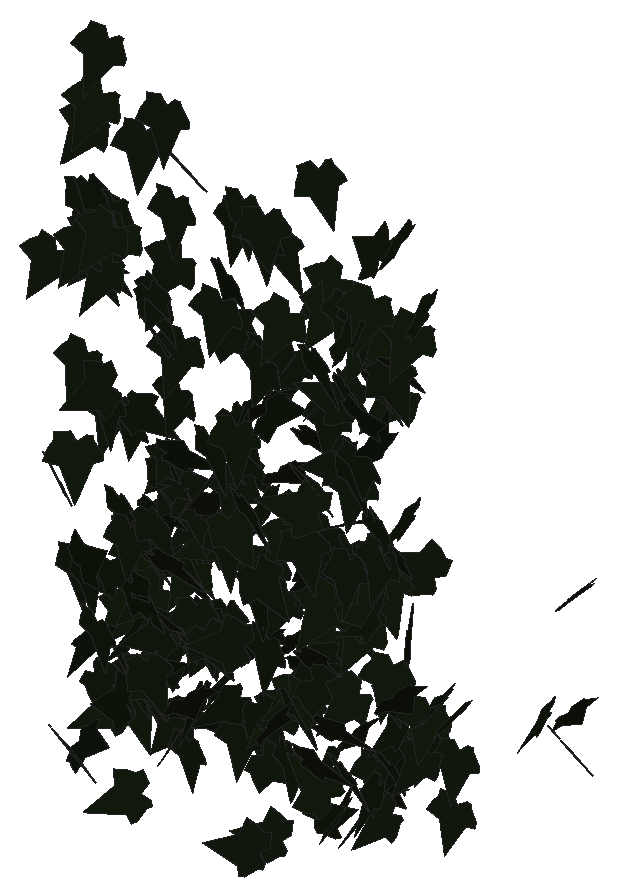
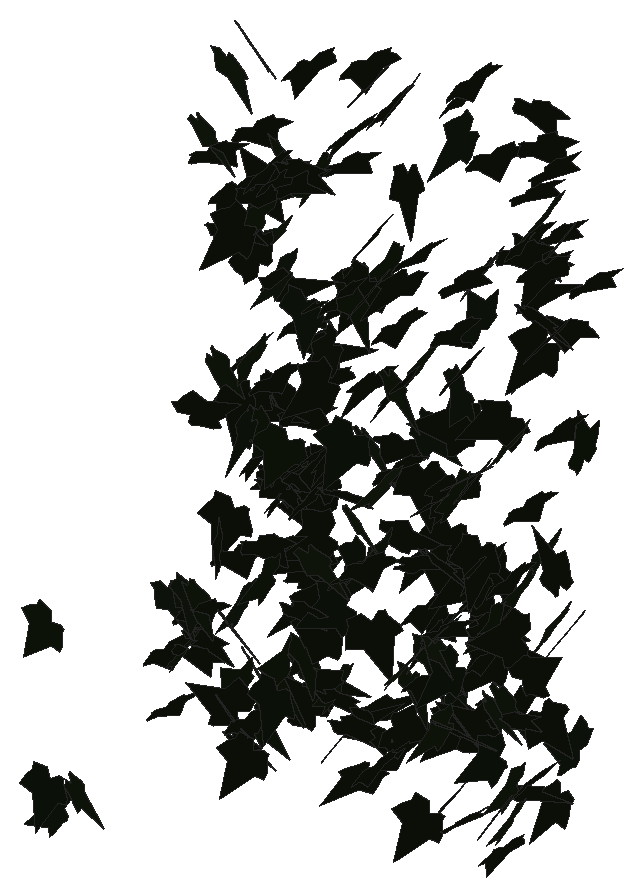
# SketchUp Ruby script. Lengths in inches.
U = 1.inch
M = Sketchup.active_model
def pt(a) = Geom::Point3d.new(a.map { |v| v * U })
def face(e, loops, mat)
  f = e.add_face(loops[0].map { |a| pt(a) })
  loops[1..].each { |l| e.add_face(l.map { |a| pt(a) }).erase! }
  f.material = f.back_material = mat if mat
  f
end
# faces: each face lists its corners as indices into pts; further lists are holes
def faces(e, pts, list, mat = nil) = list.each { |f| face(e, (f[0].is_a?(Array) ? f : [f]).map { |l| l.map { |i| pts[i] } }, mat) }
# xy, xz, yz: faces in a plane at the given z, y or x. An outline is a flat list of corners, or four numbers for a rectangle; further outlines are holes
def ring(l) = l.size == 4 ? [[l[0], l[1]], [l[2], l[1]], [l[2], l[3]], [l[0], l[3]]] : l.each_slice(2).to_a
def flat(e, list, mat, &to3) = list.each { |f| face(e, (f[0].is_a?(Array) ? f : [f]).map { |l| ring(l).map { |u, v| to3.(u, v) } }, mat) }
def xy(e, z, list, mat = nil) = flat(e, list, mat) { |x, y| [x, y, z] }
def xz(e, y, list, mat = nil) = flat(e, list, mat) { |x, z| [x, y, z] }
def yz(e, x, list, mat = nil) = flat(e, list, mat) { |y, z| [x, y, z] }
def lines(e, pts, list) = list.each { |a, b| e.add_line(pt(pts[a]), pt(pts[b])) }
# prism: a flat outline (further loops are holes) pulled along v
def prism(e, loops, v, mat = nil)
  f = face(e, loops, mat); d = Geom::Vector3d.new(v.map { |x| x * U })
  f.pushpull(f.normal.samedirection?(d) ? d.length : -d.length)
end
def box(e, o, s, mat = nil) = prism(e, [[o, [o[0] + s[0], o[1], o[2]], [o[0] + s[0], o[1] + s[1], o[2]], [o[0], o[1] + s[1], o[2]]]], [0, 0, s[2]], mat)
def at(x, y, z, deg = 0) = Geom::Transformation.translation(pt([x, y, z])) * Geom::Transformation.rotation(ORIGIN, Z_AXIS, deg.degrees)
def axes(o, x, y, z) = Geom::Transformation.new([*x, 0, *y, 0, *z, 0, *pt(o).to_a, 1])
def part(name) = M.definitions.add(name)
# library, detail: a bought-in or finely detailed component or shape, given as its bounding box
def library(name, o, s) = part(name).tap { |d| box(d.entities, o, s) }
def detail(e, o, s) = box(e.add_group.entities, o, s)
def put(e, d, t, mat = nil) = e.add_instance(d, t).tap { |i| i.material = mat if mat }
def group(e, t, mat = nil) = e.add_group.tap { |g| g.transformation = t; g.material = mat if mat }.entities
root = M.entities
M.materials.add("efeu1").color = [18, 25, 13]
c1 = part("ivyleaf_9")
p = [[1.54,2.16,1.25],[1.36,2.04,1.19],[-0.21,0.99,0.68],[-0.71,1.11,0.82],[-0.85,0.86,0.67],[-0.8,0.17,0.21],
  [-0.9,-0.01,0.1],[-0.67,-0.16,-0.02],[-0.08,-0.08,-0.05],[-0.03,-0.6,-0.4],[0.65,-0.88,-0.66],[0.83,-0.6,-0.49],
  [1.29,-0.42,-0.43],[1.8125,-0.07,-0.26],[1.21,0.44,0.15]]
faces(c1.entities,p,[[0,1,2,3,4,5,6,7,8,9,10,11,12,13,14]],"efeu1")
put(root,c1,axes([626.05,112.71,371.45],[-0.67145,-1.20045,0.4815],[-0.06051,-0.51277,-1.36278],[1.292,-0.64789,0.18641]))
put(root,c1,axes([625.96,116.39,361.48],[-0.4037,-1.34636,0.39865],[-0.06914,-0.39523,-1.40485],[1.40244,-0.40704,0.04549]))
put(root,c1,axes([625.64,121.35,333.53],[0.81653,-1.05267,-0.13594],[-0.05536,0.12904,-1.33177],[1.05997,0.81765,0.03517]))
put(root,c1,axes([625.7,117.2,369.35],[0.70417,-1.21921,-0.41464],[-0.01473,0.46492,-1.39208],[1.2877,0.67203,0.21082]))
put(root,c1,axes([627.29,117.98,342.52],[0.198,-0.141,1.37987],[-1.18466,0.70779,0.24232],[-0.72144,-1.20094,-0.01919]))
put(root,c1,axes([625.77,115.38,345.34],[0.39319,-1.37533,0.27106],[0.07663,-0.26001,-1.43043],[1.39969,0.40058,0.00217]))
put(root,c1,axes([626.96,116.38,339.04],[-0.2335,0.83704,-1.05981],[0.22412,-1.03661,-0.86809],[-1.33177,-0.3212,0.03973]))
put(root,c1,axes([626.17,117.28,368.65],[1.39761,0.45178,-0.09469],[-0.09171,-0.02413,-1.46881],[-0.45239,1.40061,0.00524]))
put(root,c1,axes([626.47,118.94,356.64],[-0.34395,-1.37252,0.18283],[-0.05405,-0.17494,-1.41493],[1.38359,-0.34803,-0.00983]))
put(root,c1,axes([626.31,121.45,331.08],[0.23264,-1.24833,-0.40414],[0.02751,0.415,-1.26602],[1.31184,0.21267,0.09822]))
put(root,c1,axes([627.52,117.14,370.7],[-1.4735,-0.05512,-0.05772],[0.0613,-0.09832,-1.4711],[0.0511,-1.47135,0.10047]))
put(root,c1,axes([627.05,117.35,387.1],[-1.22917,-0.72135,-0.37924],[0.32497,0.19554,-1.4252],[0.74737,-1.2714,-0.00403]))
put(root,c1,axes([626.3,117.21,335.16],[0.83566,-0.82721,-0.74649],[-0.12031,0.86066,-1.08841],[1.10772,0.71753,0.44493]))
put(root,c1,axes([626.32,120.25,335.4375],[1.06575,-0.85983,-0.0985],[-0.07346,0.06581,-1.36935],[0.86233,1.06827,0.00508]))
put(root,c1,axes([627.13,115.77,381.24],[-0.65135,-1.15831,0.65192],[-0.18119,-0.64184,-1.32142],[1.31676,-0.66129,0.14065]))
put(root,c1,axes([626.42,115.38,375.57],[0.58659,-1.39175,0.06191],[0.02447,-0.05687,-1.51032],[1.39292,0.5871,0.00046]))
put(root,c1,axes([626.68,116.37,374.22],[0.14066,-1.15782,-0.88511],[-0.07596,0.88219,-1.16607],[1.4554,0.15794,0.02468]))
put(root,c1,axes([627.53,119.82,340.03],[-1.08754,-0.82835,0.23481],[-0.04887,-0.31829,-1.34921],[0.8596,-1.0661,0.22037]))
put(root,c1,axes([627.47,113.97,331.47],[-0.03926,0.02081,-1.39293],[-0.76709,1.16288,0.03899],[1.16287,0.7678,-0.0213]))
put(root,c1,axes([626.71,121.72,333.64],[0.58672,-1.21149,-0.08961],[-0.05131,0.07471,-1.34602],[1.21372,0.5888,-0.01359]))
put(root,c1,axes([626.27,119.85,346.82],[1.18693,-0.31127,0.79352],[0.75843,-0.23523,-1.22671],[0.38903,1.40824,-0.02951]))
put(root,c1,axes([627.62,116,383.38],[-1.02712,-1.1019,0.00701],[-0.02789,0.01642,-1.50604],[1.10157,-1.02702,-0.0316]))
put(root,c1,axes([628.29,117.54,333.05],[-1.1996,-0.27111,0.6453],[-0.54996,-0.42696,-1.20174],[0.43296,-1.2935,0.26142]))
put(root,c1,axes([628.3,120.58,341.22],[-1.15049,0.45272,-0.54823],[0.43215,-0.38285,-1.22304],[-0.56459,-1.21557,0.18102]))
put(root,c1,axes([627.27,114.84,345.05],[0.37798,-1.26334,0.48366],[0.14913,-0.46021,-1.31864],[1.34452,0.4062,0.01029]))
put(root,c1,axes([627.37,118.41,349.22],[0.64063,-1.21051,0.35995],[0.16692,-0.31891,-1.36958],[1.25181,0.66202,-0.00158]))
put(root,c1,axes([628.26,115.17,372.93],[-0.69581,-1.09577,0.67655],[-0.16852,-0.6849,-1.28261],[1.27672,-0.68759,0.19942]))
put(root,c1,axes([627.93,120.16,337.06],[1.29444,-0.24286,0.25292],[0.24253,-0.07849,-1.31664],[0.25324,1.31658,-0.03184]))
put(root,c1,axes([628.16,114.17,377.01],[0.90407,-1.16045,-0.26707],[-0.08156,0.27419,-1.46747],[1.18799,0.90194,0.1025]))
put(root,c1,axes([628.84,119.23,345.84],[-0.71,-1.10406,-0.33576],[0.36371,0.16003,-1.29534],[1.09517,-0.76891,0.21251]))
put(root,c1,axes([630.01,117.11,340.04],[-1.02088,0.95691,-0.16624],[0.10553,-0.13047,-1.39906],[-0.9655,-1.02607,0.02286]))
put(root,c1,axes([629.05,115.66,375.1],[-0.11695,-1.44613,0.25942],[-0.03601,-0.25734,-1.45078],[1.46878,-0.12146,-0.01491]))
put(root,c1,axes([629.54,112.14,373.77],[-0.67362,-1.19407,0.51458],[-0.08169,-0.53952,-1.35889],[1.29765,-0.65381,0.18157]))
put(root,c1,axes([628.52,110.67,333.26],[0.84672,-0.92304,0.76005],[0.58924,-0.48827,-1.24941],[1.04043,1.02772,0.08904]))
put(root,c1,axes([628.84,112.33,347.07],[-0.16438,0.13905,1.47625],[0.91408,-1.15999,0.21104],[1.16752,0.92777,0.04261]))
put(root,c1,axes([628.95,109.42,355.53],[-0.027,-0.57991,1.37103],[0.55583,-1.27601,-0.52878],[1.38097,0.50224,0.23963]))
put(root,c1,axes([629.24,119.5625,344.44],[0.16291,-1.35705,-0.09852],[-0.01392,0.09755,-1.36679],[1.36055,0.16349,-0.00219]))
put(root,c1,axes([629.04,118.39,346.44],[1.20901,-0.69536,-0.09625],[-0.04936,0.10701,-1.39306],[0.70025,1.20811,0.06799]))
put(root,c1,axes([630.15,115.24,373.71],[-0.90624,-1.171,0.03617],[-0.00741,-0.04,-1.48059],[1.17153,-0.90608,0.01862]))
put(root,c1,axes([630.01,116.43,348.6],[-0.04433,-1.39838,0.16525],[-0.01018,-0.16501,-1.39908],[1.40808,-0.04522,-0.00491]))
put(root,c1,axes([631.61,121.4,338.7],[-1.2008,0.3892,0.4893],[-0.57162,-0.25428,-1.20059],[-0.25325,-1.27149,0.38988]))
put(root,c1,axes([630.72,121.08,331.28],[-0.65416,-0.97894,0.63666],[-0.01251,-0.72384,-1.12583],[1.1677,-0.55617,0.34461]))
put(root,c1,axes([631.49,112.21,372.64],[-1.39977,-0.3276,-0.31618],[0.30187,0.09743,-1.43737],[0.34083,-1.43173,-0.02547]))
put(root,c1,axes([630.61,115.66,358.31],[0.0882,-1.21713,0.73176],[0.24167,-0.70961,-1.20942],[1.39945,0.19925,0.16273]))
put(root,c1,axes([630.8,116.65,342.45],[1.36908,0.29321,0.06626],[0.06288,0.0228,-1.4001],[-0.29396,1.3705,0.00911]))
put(root,c1,axes([631.31,116.49,381.37],[-0.48296,-1.40463,-0.19776],[0.06922,0.18533,-1.48534],[1.4168,-0.48787,0.00515]))
put(root,c1,axes([631.66,113.83,336.06],[-0.18668,-0.20118,1.47783],[-0.64595,-1.33152,-0.26286],[1.34432,-0.66774,0.07891]))
put(root,c1,axes([631.68,117.34,350.68],[1.15815,0.45956,-0.79965],[-0.75119,-0.27475,-1.24586],[-0.53512,1.38031,0.01825]))
put(root,c1,axes([632.28,116.16,337.54],[-1.139,-0.51688,0.6399],[-0.51563,-0.40294,-1.24328],[0.64091,-1.24275,0.13696]))
put(root,c1,axes([631.09,120.96,343.3],[1.35615,0.04148,-0.09359],[-0.09411,0.01609,-1.35665],[-0.04027,1.35928,0.01892]))
put(root,c1,axes([631.32,117.05,350.0625],[0.54204,-1.16959,-0.59984],[-0.15631,0.58688,-1.28557],[1.30511,0.55604,0.09516]))
put(root,c1,axes([632.19,116.58,344.42],[-0.78438,-0.91359,0.64291],[-0.33818,-0.55451,-1.20057],[1.06471,-0.84917,0.0923]))
put(root,c1,axes([632.02,111.69,376],[-0.79372,-1.13052,0.5055],[-0.08367,-0.55009,-1.36162],[1.23556,-0.76349,0.23253]))
put(root,c1,axes([632.58,118.58,337.61],[-1.28181,0.46933,-0.21974],[0.19815,-0.09783,-1.36483],[-0.47885,-1.29683,0.02343]))
put(root,c1,axes([630.96,117.86,336.72],[0.28476,-0.25496,1.34292],[1.31194,-0.33411,-0.34163],[0.38373,1.3315,0.17142]))
put(root,c1,axes([633,120.33,343.99],[-0.74733,1.13045,0.23543],[-0.30116,0.07991,-1.33969],[-1.11475,-0.77945,0.2041]))
put(root,c1,axes([631.59,121.22,338.8],[1.23994,-0.43864,-0.32699],[-0.21776,0.34741,-1.29177],[0.5019,1.23437,0.24737]))
put(root,c1,axes([631.6875,111.63,362.31],[0.27382,-1.40281,0.24989],[0.02005,-0.25065,-1.42901],[1.42475,0.27313,-0.02792]))
put(root,c1,axes([631.49,114.57,359.95],[0.07904,-0.13601,-1.43122],[0.73177,1.23761,-0.07719],[1.2375,-0.72315,0.13706]))
put(root,c1,axes([632.1,120.06,346.07],[0.76216,-1.13108,-0.30205],[0.01865,0.3721,-1.34635],[1.17056,0.73052,0.21812]))
put(root,c1,axes([632.6,121.97,331.7],[1.07493,0.7792,0.06414],[0.04499,0.04723,-1.32759],[-0.78054,1.07581,0.01182]))
put(root,c1,axes([633,120.01,345.16],[-0.76039,-1.12504,0.32421],[0.0281,-0.404,-1.33604],[1.17048,-0.72117,0.24268]))
put(root,c1,axes([633.3,117.84,371.25],[-0.70099,-1.1796,0.63665],[-0.18472,-0.62659,-1.36434],[1.32765,-0.71,0.14633]))
put(root,c1,axes([633.17,119.06,331.0625],[0.24105,-1.26746,0.4019],[0.13676,-0.38265,-1.28878],[1.3226,0.27057,0.06002]))
put(root,c1,axes([634.3,119.41,350.18],[-1.37408,-0.03381,-0.1199],[0.12285,-0.14782,-1.36626],[0.02063,-1.37136,0.15023]))
put(root,c1,axes([633.79,117.11,355.15],[-0.79722,-0.92919,0.73564],[0.00626,-0.88988,-1.11723],[1.18513,-0.62036,0.50075]))
put(root,c1,axes([633.02,115.83,347.64],[1.45478,0.05186,0.25804],[0.25802,0.00505,-1.4557],[-0.05195,1.47748,-0.00409]))
put(root,c1,axes([633.3,115.89,355.07],[0.60599,-1.28618,-0.12622],[-0.04178,0.11984,-1.42172],[1.29168,0.60728,0.01323]))
put(root,c1,axes([633.29,108.54,345.5625],[0.39647,-1.30208,0.61517],[0.24204,-0.56873,-1.35977],[1.4196,0.46061,0.06003]))
put(root,c1,axes([634.48,108.38,365.32],[-0.66363,-0.73428,1.15007],[-0.69337,-0.91998,-0.98747],[1.17518,-0.95744,0.06683]))
put(root,c1,axes([633.26,112.78,346.75],[-0.00735,-0.12223,-1.45499],[1.39647,0.42429,-0.0427],[0.42637,-1.39177,0.11476]))
put(root,c1,axes([633.95,114.7,369.95],[-0.13303,-1.10095,0.95258],[0.12613,-0.96166,-1.09384],[1.45037,-0.01735,0.1825]))
put(root,c1,axes([633.54,114.91,366.47],[0.14701,-0.85265,1.23638],[0.696,-1.06217,-0.81526],[1.33088,0.64965,0.28978]))
put(root,c1,axes([633.62,117.38,354.38],[0.9197,-1.05899,0.26601],[0.14525,-0.22605,-1.4021],[1.08218,0.93033,-0.03788]))
put(root,c1,axes([634.07,116.05,335.79],[1.05608,0.74421,0.40226],[0.3313,0.22819,-1.29195],[-0.77839,1.10682,-0.00411]))
put(root,c1,axes([634.26,104.94,362.11],[-0.80497,-1.02477,-0.70081],[0.5895,0.41957,-1.29062],[1.0926,-0.98136,0.18002]))
put(root,c1,axes([633.99,113.72,370.5],[0.7176,-1.20347,-0.40129],[-0.13829,0.38408,-1.39917],[1.26105,0.72696,0.07492]))
put(root,c1,axes([634.33,119.6,340.86],[-0.04589,-1.29505,-0.4348],[0.14961,0.42767,-1.28959],[1.35788,-0.09089,0.12739]))
put(root,c1,axes([634.41,115.3125,381.48],[1.45145,-0.18507,-0.35803],[-0.33324,0.20156,-1.45515],[0.22668,1.48131,0.15328]))
put(root,c1,axes([634.54,114.8,385.34],[-0.07405,-1.51309,0.00427],[-0.02418,-0.00309,-1.51471],[1.5129,-0.07411,-0.024]))
put(root,c1,axes([633.97,113.27,344.68],[0.70089,-0.52509,1.12204],[0.95647,-0.58995,-0.87355],[0.78732,1.18414,0.06234]))
put(root,c1,axes([634.9,115.91,354.22],[0.02363,-1.06706,-1.07303],[-0.06346,1.07152,-1.06695],[1.51195,0.06165,-0.02801]))
put(root,c1,axes([636.05,117.53,341.58],[-0.6103,1.25574,0.27902],[-0.09761,0.26274,-1.39594],[-1.28265,-0.61749,-0.02653]))
put(root,c1,axes([635.22,115.81,366.01],[-0.55727,-1.37609,0.09712],[-0.0065,-0.10213,-1.4843],[1.3795,-0.55638,0.03224]))
put(root,c1,axes([635.93,113.79,360.1],[0.00485,0.97409,1.11854],[-0.01609,1.11851,-0.974],[-1.48315,-0.00895,0.01422]))
put(root,c1,axes([635.98,113.16,343.55],[-0.47809,-0.47412,1.20223],[-0.82187,-0.87769,-0.67297],[0.99732,-0.95057,0.02174]))
put(root,c1,axes([635.375,117.0625,343.36],[0.7135,-0.75192,-0.96683],[-0.46365,0.86984,-1.01865],[1.13366,0.82899,0.19189]))
put(root,c1,axes([635.32,115.33,362.2],[-0.10027,-1.29004,0.74225],[0.03537,-0.74578,-1.29141],[1.48791,-0.06921,0.08072]))
put(root,c1,axes([636.51,119.23,348.74],[-1.1409,-0.2832,0.78427],[-0.62821,-0.58206,-1.12405],[0.5483,-1.25616,0.34404]))
put(root,c1,axes([635.26,120.96,341.94],[0.57907,-1.24001,-0.0136],[0.10572,0.06432,-1.36302],[1.23557,0.57565,0.123]))
put(root,c1,axes([635.49,111.47,341.7],[-0.49708,-0.56739,-1.25746],[1.09852,0.64572,-0.72562],[0.8345,-1.188,0.20617]))
put(root,c1,axes([636.67,112.72,334.88],[-0.68634,1.03083,-0.83423],[-0.52186,0.65359,1.23697],[1.2191,0.86013,0.05985]))
put(root,c1,axes([635.85,116.73,352.79],[0.03452,-1.43734,-0.0753],[0.3114,0.081,-1.40331],[1.40523,0.01736,0.31282]))
put(root,c1,axes([635.35,114.24,357.65],[1.02681,-0.1813,1.04982],[1.04722,-0.09613,-1.04087],[0.19575,1.46534,0.06161]))
put(root,c1,axes([636.21,116.62,341.53],[-0.18748,-1.10272,0.87642],[0.23614,-0.89624,-1.07714],[1.38864,0.00353,0.30149]))
put(root,c1,axes([637.22,119.62,335.9],[-0.21647,-0.18922,-1.32688],[0.21514,-1.33155,0.15479],[-1.32292,-0.18558,0.24229]))
put(root,c1,axes([637.54,116.18,354.19],[0.22378,1.27383,-0.53827],[-0.03765,-0.53946,-1.2923],[-1.38238,0.2209,-0.05194]))
put(root,c1,axes([637.93,116.87,338.34],[-0.54975,1.19055,0.39748],[-0.16053,0.36368,-1.31134],[-1.24485,-0.57267,-0.00643]))
put(root,c1,axes([637.1875,116.32,343.96],[-0.02784,-1.40594,-0.24864],[-0.01802,0.24901,-1.40603],[1.42764,-0.02427,-0.0226]))
put(root,c1,axes([637.52,119.72,333.5],[-0.11257,-1.34264,0.15888],[0.01602,-0.16074,-1.34704],[1.35192,-0.10989,0.02919]))
put(root,c1,axes([637.47,121.625,333.65],[0.14232,-1.32639,-0.08879],[0.0164,0.09104,-1.33375],[1.32925,0.14089,0.02596]))
put(root,c1,axes([637.61,114.4,345.75],[-0.81826,-0.68227,-0.87434],[0.83758,0.33202,-1.04295],[0.72693,-1.15056,0.21751]))
put(root,c1,axes([637.47,120.17,355.08],[0.98225,-0.96205,-0.2297],[0.06741,0.38808,-1.33715],[0.98679,0.93111,0.31998]))
put(root,c1,axes([638.95,114.4375,356.67],[-0.91493,0.72344,-0.81171],[0.3584,-0.80089,-1.11779],[-1.02654,-0.92441,0.33319]))
put(root,c1,axes([639.43,105.57,335.05],[-1.15272,-0.25774,0.753],[-0.69714,-0.31242,-1.17414],[0.38398,-1.34096,0.12883]))
put(root,c1,axes([638.61,118.06,354.95],[-0.4364,-1.35508,0.15136],[0.01176,-0.16266,-1.42233],[1.36346,-0.43231,0.06072]))
put(root,c1,axes([638.65,110.65,380.93],[0.06661,-1.47178,0.27933],[0.04232,-0.27765,-1.473],[1.49746,0.07331,0.0292]))
put(root,c1,axes([638.78,115.73,370.46],[-0.29218,-1.40869,0.33526],[0.13029,-0.36621,-1.42516],[1.44216,-0.25232,0.19667]))
put(root,c1,axes([639.87,116.77,360.91],[-0.96783,1.04536,-0.08556],[0.06226,-0.05896,-1.42459],[-1.04701,-0.96981,-0.00562]))
put(root,c1,axes([640.14,118.53,342.51],[0.12869,1.19937,-0.75286],[-0.29422,-0.71682,-1.19225],[-1.38518,0.26369,0.18329]))
put(root,c1,axes([639.05,116.79,360.87],[0.70045,-1.11799,-0.5801],[-0.17858,0.56892,-1.31206],[1.24681,0.70956,0.13797]))
put(root,c1,axes([638.87,120.01,335.67],[-0.14844,-0.47476,-1.3209],[1.20797,0.63324,-0.36335],[0.71483,-1.16869,0.33972]))
put(root,c1,axes([639.27,116.02,368.74],[0.51987,-0.7931,-1.17638],[-0.12061,1.22363,-0.87826],[1.41363,0.39606,0.35769]))
put(root,c1,axes([639.67,120.02,347.95],[-0.50509,-1.29081,-0.17502],[0.03743,0.17326,-1.38583],[1.30208,-0.5057,-0.02806]))
put(root,c1,axes([639.84,112.125,340.71],[-0.46153,0.45942,-1.23349],[0.88896,-0.85518,-0.65114],[-0.97072,-1.00158,-0.00983]))
put(root,c1,axes([640.46,121.1,335.76],[-1.24787,-0.53442,0.11195],[-0.10382,-0.04195,-1.35749],[0.53605,-1.25218,-0.0023]))
put(root,c1,axes([639.45,120.01,331.78],[0.4004,-0.5492,-1.21421],[0.06794,1.2746,-0.55411],[1.33091,0.10016,0.39358]))
put(root,c1,axes([640,112.6,345.375],[0.22161,-1.04534,-0.88327],[-0.00304,0.8944,-1.05927],[1.36854,0.17126,0.14068]))
put(root,c1,axes([639.84,113.26,360.75],[0.60065,-1.35241,0.32448],[0.14087,-0.29247,-1.47976],[1.38364,0.61687,0.0098]))
put(root,c1,axes([641.28,113.23,374.76],[0.79602,0.20162,-1.26609],[-1.26279,-0.13395,-0.81528],[-0.22131,1.48953,0.09806]))
put(root,c1,axes([640.5,114.21,352.84],[0.17706,-1.42826,0.03133],[-0.01537,-0.03347,-1.43906],[1.42852,0.17667,-0.01937]))
put(root,c1,axes([641.72,118.9375,350.65],[-1.1939,0.72043,-0.06653],[0.05756,-0.0334,-1.39442],[-0.72121,-1.19528,-0.00114]))
put(root,c1,axes([641.81,121.1,337.46],[-1.31424,-0.3388,0.11687],[-0.08247,-0.14642,-1.35182],[0.34877,-1.31128,0.12075]))
put(root,c1,axes([641.01,117.1875,346.55],[0.31711,-1.16478,0.83285],[0.27379,-0.78797,-1.20626],[1.40549,0.4163,0.04706]))
put(root,c1,axes([641.16,113.86,354.35],[-0.25789,-0.96763,-0.97719],[0.70895,0.75838,-0.93807],[1.17839,-0.66803,0.35051]))
put(root,c1,axes([641.88,118.67,356.51],[0.78806,1.18306,0.22995],[0.01987,0.26195,-1.41582],[-1.20504,0.778,0.12703]))
put(root,c1,axes([641.71,119.49,346.2],[-0.38234,-1.23702,0.49471],[0.00056,-0.51483,-1.28689],[1.33228,-0.35479,0.14251]))
put(root,c1,axes([642.83,115.99,355.09],[-1.04259,0.98196,0.09227],[-0.07033,0.05992,-1.43221],[-0.98378,-1.04495,0.00459]))
put(root,c1,axes([641.65,117.125,367.11],[0.3003,-1.40547,0.3462],[0.07035,-0.33898,-1.43719],[1.44577,0.30843,-0.00198]))
put(root,c1,axes([643.35,112.28,345.56],[-0.95572,0.01019,1.01738],[-1.01739,0.00189,-0.95576],[-0.00835,-1.39587,0.00613]))
put(root,c1,axes([642.0625,114.27,380.46],[0.23384,-1.47474,0.17437],[0.06655,-0.16594,-1.49265],[1.48353,0.2399,0.03947]))
put(root,c1,axes([642.89,106.62,343.57],[0.39505,1.35802,-0.05307],[-0.01682,-0.05038,-1.41432],[-1.35896,0.39541,0.00208]))
put(root,c1,axes([643.5,120.39,337.6875],[-1.10211,-0.34591,0.71878],[-0.69475,-0.18611,-1.15483],[0.39195,-1.30255,-0.02588]))
put(root,c1,axes([641.96,119.8,337.53],[0.89555,-1.06528,0.12002],[0.08213,-0.08776,-1.39168],[1.06887,0.89928,0.00637]))
put(root,c1,axes([642.24,119.67,332.98],[0.15927,-1.22228,0.55434],[0.08031,-0.54855,-1.23259],[1.33971,0.1782,0.00799]))
put(root,c1,axes([643.04,118.84,351.91],[-1.26698,-0.65815,-0.08821],[0.27322,-0.34349,-1.36145],[0.60523,-1.22271,0.42994]))
put(root,c1,axes([642.45,112.97,362.6875],[-0.06666,-1.45743,-0.11975],[-0.01477,0.12054,-1.45882],[1.46227,-0.06522,-0.02019]))
put(root,c1,axes([643.63,116.4,366.04],[-0.6218,1.2979,0.10009],[-0.04569,0.08909,-1.43916],[-1.30095,-0.62347,0.00271]))
put(root,c1,axes([642.42,113.01,379.92],[0.11495,-1.31351,0.72253],[0.05021,-0.72087,-1.31848],[1.49828,0.12493,-0.01125]))
put(root,c1,axes([642.77,118.37,342.9],[0.76861,0.64431,0.97009],[0.49729,0.86944,-0.97147],[-1.05305,0.88086,0.2493]))
put(root,c1,axes([643.9,121.1875,340.24],[-0.4328,1.19139,0.5005],[-0.14252,0.4806,-1.26725],[-1.28437,-0.4548,-0.02803]))
put(root,c1,axes([644.25,120.11,347.09],[-0.92489,1.02033,-0.07781],[-0.24858,-0.32576,-1.31705],[-0.99264,-0.86911,0.40232]))
put(root,c1,axes([643.26,119.57,341.35],[1.20282,0.71154,0.09584],[0.07878,0.05507,-1.39751],[-0.71363,1.20538,0.00727]))
put(root,c1,axes([643.39,118.27,366.79],[-0.11908,-1.3992,0.28998],[-0.0357,-0.28798,-1.40421],[1.42848,-0.12383,-0.01092]))
put(root,c1,axes([643.5,118.54,354.9],[0.54223,-1.19375,-0.50297],[-0.20992,0.45708,-1.31112],[1.27826,0.58144,-0.00196]))
put(root,c1,axes([643.5,115.15,344.73],[0.14265,-1.39849,0.51335],[0.01174,-0.51462,-1.40523],[1.48968,0.13797,-0.03809]))
put(root,c1,axes([644.75,121.11,343.28],[-1.30832,-0.40066,-0.0487],[0.05165,-0.00236,-1.36818],[0.40029,-1.30922,0.01737]))
put(root,c1,axes([643.87,118.93,360.24],[1.4104,0.09144,0.13178],[0.13081,0.01925,-1.41332],[-0.09283,1.41641,0.0107]))
put(root,c1,axes([644.63,113.43,365.34],[0.65132,1.2331,0.39354],[0.19488,0.34211,-1.39449],[-1.27962,0.67974,-0.01207]))
put(root,c1,axes([644.57,113.53,368.54],[-0.06362,-1.23456,0.76645],[0.04728,-0.76853,-1.234],[1.45236,-0.02906,0.07375]))
put(root,c1,axes([645.88,110.98,330.2],[-0.69516,0.07354,1.22552],[-1.04205,-0.78002,-0.54428],[0.64918,-1.17333,0.43864]))
put(root,c1,axes([644.55,114.98,378.04],[0.48171,-1.36019,-0.41762],[0.08258,0.46688,-1.4254],[1.42046,0.43413,0.22449]))
put(root,c1,axes([645.95,113.49,330.16],[-0.58002,0.03341,1.20078],[-0.99113,-0.76671,-0.45742],[0.67871,-1.09108,0.3582]))
put(root,c1,axes([645.34,112.97,365.05],[0.01359,0.2771,-1.43012],[-0.62081,1.2949,0.245],[1.3178,0.60716,0.13016]))
put(root,c1,axes([645.46,118.01,342.62],[0.49446,-0.46832,-1.33611],[-0.20165,1.37753,-0.55746],[1.40138,0.36346,0.39121]))
put(root,c1,axes([645.32,112.34,380.07],[0.20484,-1.42348,0.43015],[0.19636,-0.40452,-1.43216],[1.47403,0.2517,0.13101]))
put(root,c1,axes([645.88,111.875,381.52],[-0.27334,-1.42749,-0.37313],[0.03756,0.37263,-1.45307],[1.47498,-0.27403,-0.03215]))
put(root,c1,axes([646.04,119.03,353.03],[-0.32865,-1.25379,0.59137],[0.08841,-0.62548,-1.27698],[1.38343,-0.25788,0.22209]))
put(root,c1,axes([645.98,118.48,350.125],[-0.04114,-1.28781,0.54306],[-0.01022,-0.543,-1.28845],[1.39759,-0.04188,0.00656]))
put(root,c1,axes([646.9,117.29,364.625],[-0.0597,1.38799,0.42023],[-0.11165,0.41494,-1.38637],[-1.4459,-0.08935,0.08971]))
put(root,c1,axes([646.78,120.6875,335.71],[0.16167,1.31464,0.37443],[0.04927,0.37119,-1.32454],[-1.36603,0.16897,-0.00346]))
put(root,c1,axes([646.29,115.39,350.73],[0.46661,0.56571,1.22616],[0.5926,1.07992,-0.72375],[-1.21339,0.74496,0.11806]))
put(root,c1,axes([647.12,112.96,373.64],[-0.77472,-1.21466,0.2883],[-0.01241,-0.33179,-1.43125],[1.24834,-0.75712,0.16469]))
put(root,c1,axes([646.74,117.02,383.43],[0.07665,-1.36024,-0.57767],[-0.02079,0.5774,-1.36235],[1.47768,0.07868,0.0108]))
put(root,c1,axes([647.47,110.27,341.25],[0.23398,1.12059,0.81922],[0.21968,0.79041,-1.14393],[-1.37061,0.31799,-0.04349]))
put(root,c1,axes([647.53,118.63,354.18],[0.76176,1.16442,0.23272],[-0.34018,0.4789,-1.28267],[-1.13767,0.63647,0.53936]))
put(root,c1,axes([647,118.02,363.72],[-0.06065,-1.44042,0.20084],[-0.01815,-0.20025,-1.44166],[1.45424,-0.06258,-0.00962]))
put(root,c1,axes([648.21,116.43,335.61],[-1.01455,0.86091,0.11384],[-0.10399,0.05336,-1.33033],[-0.86216,-1.01952,0.0265]))
put(root,c1,axes([646.94,114.46,359.97],[1.41556,-0.23149,-0.35118],[-0.34133,0.08821,-1.43402],[0.24577,1.4558,0.03105]))
put(root,c1,axes([648.2,117.3125,374.95],[-1.37283,-0.5316,0.11045],[-0.07743,-0.10556,-1.47049],[0.53741,-1.37322,0.07028]))
put(root,c1,axes([647.54,119.39,351.9375],[-0.98496,-0.72047,-0.66921],[0.57458,0.34699,-1.21923],[0.79799,-1.13912,0.05187]))
put(root,c1,axes([649.06,117.5,365.04],[-0.5457,0.23019,1.33071],[-1.35043,-0.10494,-0.53563],[0.01123,-1.43442,0.25274]))
put(root,c1,axes([647.35,120.59,344.5625],[1.111,-0.81319,-0.04385],[-0.02498,0.0401,-1.3767],[0.81399,1.11114,0.01759]))
put(root,c1,axes([647.91,122,331.21],[1.02429,0.80989,0.06334],[-0.01068,0.11535,-1.30218],[-0.81229,1.01974,0.09699]))
put(root,c1,axes([649.3125,113.26,358.12],[-0.71735,0.11468,1.30667],[-1.30858,-0.16508,-0.70391],[0.09029,-1.48146,0.17958]))
put(root,c1,axes([647.26,114.75,345.21],[1.43279,-0.13266,0.43871],[0.4356,-0.05363,-1.43886],[0.14253,1.49749,-0.01267]))
put(root,c1,axes([648.32,116.85,373.36],[-0.75432,-1.20456,0.40338],[-0.143,-0.38564,-1.41898],[1.26223,-0.76354,0.0803]))
put(root,c1,axes([647.76,108.68,354.82],[0.46166,-1.10277,-0.88458],[-0.09736,0.90355,-1.17722],[1.41036,0.42335,0.20829]))
put(root,c1,axes([647.54,119.23,351.25],[-0.32669,-0.5384,-1.24007],[1.19155,0.48799,-0.52578],[0.63863,-1.1859,0.34664]))
put(root,c1,axes([648.44,121.85,333.6],[-0.35812,-1.28837,-0.09768],[0.03193,0.0925,-1.33721],[1.29168,-0.35949,0.00597]))
put(root,c1,axes([647.63,115.57,331.63],[0.08496,-0.10711,1.45815],[1.29107,-0.67996,-0.12518],[0.68615,1.2927,0.05498]))
put(root,c1,axes([648.32,117.59,349.84],[0.55702,-1.30764,-0.24104],[-0.07208,0.23126,-1.42113],[1.32771,0.56115,0.02397]))
put(root,c1,axes([649.08,119.67,346.21],[-1.01138,-0.96557,-0.03006],[0.02616,0.01613,-1.39827],[0.96568,-1.01169,0.0064]))
put(root,c1,axes([648.37,117.54,366.74],[1.20728,-0.795,-0.27537],[-0.16937,0.24211,-1.44155],[0.82412,1.21438,0.10713]))
put(root,c1,axes([648.37,114.4375,343.55],[0.30687,-0.21667,-1.432],[0.39468,1.4209,-0.13042],[1.39348,-0.35473,0.35229]))
put(root,c1,axes([648.95,118.52,358.66],[-0.31623,-1.40158,0.10554],[0.0073,-0.10981,-1.43647],[1.40552,-0.31477,0.0312]))
put(root,c1,axes([648.8,112.64,356.09],[-0.08445,-1.33017,-0.49594],[0.1387,0.48671,-1.32903],[1.41282,-0.12729,0.10083]))
put(root,c1,axes([649.77,114.95,332.25],[-0.88006,0.88712,-0.84277],[-0.58681,0.60496,1.24957],[1.07373,1.05773,-0.00785]))
put(root,c1,axes([648.4,106.1875,361.84],[0.9733,-1.07747,0.38027],[0.23851,-0.29694,-1.45183],[1.11744,1.00187,-0.02133]))
put(root,c1,axes([649.89,118.74,331.78],[-0.93348,0.69519,-0.62259],[0.37705,-0.52456,-1.15107],[-0.85366,-0.99189,0.17239]))
put(root,c1,axes([648.85,116.84,335.66],[0.89342,-0.95047,0.46252],[0.336,-0.31882,-1.30421],[1.0022,0.95419,0.02494]))
put(root,c1,axes([649.61,117.02,373.33],[-0.2801,-1.41745,0.3331],[0.04074,-0.3467,-1.44108],[1.45549,-0.26307,0.10444]))
put(root,c1,axes([650.52,120.39,330.78],[-1.31805,-0.07378,0.01667],[-0.01261,-0.07241,-1.31817],[0.07458,-1.31617,0.07158]))
put(root,c1,axes([650.52,121.94,334.32],[-1.18305,0.52033,-0.24498],[0.21572,-0.11794,-1.29225],[-0.53312,-1.20237,0.02074]))
put(root,c1,axes([650.37,116.9375,353.35],[0.19297,0.87488,1.10872],[-0.07965,1.12398,-0.87306],[-1.41008,0.05624,0.20105]))
put(root,c1,axes([649.27,122.05,334.06],[0.02553,-0.00082,1.33622],[1.33267,0.09732,-0.0254],[-0.09729,1.33291,0.00268]))
put(root,c1,axes([650.1,119.4,355.02],[1.16052,-0.3505,-0.70777],[-0.67365,0.21742,-1.21224],[0.4123,1.34182,0.01154]))
put(root,c1,axes([651.43,113.74,362.84],[-1.05604,0.85098,0.45147],[-0.57391,-0.01773,-1.30902],[-0.7737,-1.14836,0.35477]))
put(root,c1,axes([649.72,112.5,371.41],[0.93339,-1.1679,0.18815],[0.1263,-0.13991,-1.49502],[1.1762,0.94183,0.01122]))
put(root,c1,axes([650.1875,118.08,352.2],[0.42587,-1.31597,-0.25207],[-0.11138,0.22881,-1.38272],[1.33525,0.43881,-0.03495]))
put(root,c1,axes([650.33,119.62,341.21],[1.04049,-0.90144,-0.2105],[-0.15409,0.1436,-1.37664],[0.91277,1.05181,0.00755]))
put(root,c1,axes([650.61,117.08,373.69],[0.11907,-1.47073,0.13778],[-0.03043,-0.14064,-1.47496],[1.47685,0.11568,-0.0415]))
put(root,c1,axes([650.25,120.61,334.67],[0.30819,-0.96206,0.9269],[0.60478,-0.74771,-0.97716],[1.19119,0.62853,0.25631]))
put(root,c1,axes([651.33,117.31,371.85],[-1.14366,-0.89017,-0.15094],[0.1067,0.10863,-1.44912],[0.89655,-1.14845,-0.02008]))
put(root,c1,axes([651.6875,112.28,352.23],[-1.05865,-1.039,0.20658],[-0.1267,-0.16577,-1.48304],[1.05173,-1.0658,0.02928]))
put(root,c1,axes([652.1875,119.56,339.13],[-1.24857,0.51279,-0.12514],[0.11168,-0.05745,-1.34973],[-0.51589,-1.25351,0.01067]))
put(root,c1,axes([651.83,117.21,334.88],[-1.11198,0.14756,-0.71953],[0.69529,-0.20943,-1.11746],[-0.2368,-1.30781,0.09776]))
put(root,c1,axes([650.78,117.16,370.11],[0.9545,-1.06604,0.38231],[0.40501,-0.14562,-1.4172],[1.05763,1.01785,0.19767]))
put(root,c1,axes([652.5,113.04,373],[-1.15984,0.66073,-0.71144],[-0.61642,0.35523,1.33483],[0.75016,1.31346,-0.00312]))
put(root,c1,axes([652.26,120.11,344.42],[-0.01188,-0.19475,1.38092],[0.05064,1.38,0.19506],[-1.39366,0.0518,-0.00468]))
put(root,c1,axes([652.57,135.64,333.01],[-1.01612,0.67049,-0.50136],[0.34457,-0.38364,-1.21141],[-0.76302,-1.06615,0.12061]))
put(root,c1,axes([651.98,118.72,344.03],[-0.63013,-1.22041,-0.21851],[0.10045,0.19405,-1.37348],[1.23574,-0.63808,0.00023]))
put(root,c1,axes([652.98,110.15,337.7],[-0.97382,-1.02651,-0.21507],[-0.14229,-0.16146,1.41492],[-1.0391,0.98413,0.0078]))
put(root,c1,axes([651.74,118.25,369.38],[1.41874,0.26826,0.01661],[0.01597,0.00496,-1.44388],[-0.2683,1.41883,0.0019]))
put(root,c1,axes([652.15,113.66,354.9],[-1.08942,-0.34015,-0.8981],[0.85067,0.28851,-1.14115],[0.4457,-1.38209,-0.01719]))
put(root,c1,axes([652.78,115.55,375.6],[-0.71704,-1.27837,0.00389],[0.02663,-0.01939,-1.46537],[1.2781,-0.71679,0.03271]))
put(root,c1,axes([652.26,115.77,369.2],[1.25009,-0.73499,-0.26237],[-0.20351,0.17129,-1.44949],[0.75341,1.26579,0.0438]))
put(root,c1,axes([653.06,122.11,337.45],[-1.0451,-0.73248,-0.38309],[0.39909,0.09368,-1.26786],[0.72389,-1.10915,0.14591]))
put(root,c1,axes([652.32,113.38,363.17],[0.67015,-1.24736,0.22064],[0.11344,-0.18952,-1.41595],[1.26164,0.67961,0.01012]))
put(root,c1,axes([653.49,116.56,355.2],[0.91739,0.3261,-1.05216],[-1.04492,-0.17571,-0.96554],[-0.3486,1.38484,0.12525]))
put(root,c1,axes([652.66,116.03,357.3],[0.54292,-1.16136,0.64439],[0.30648,-0.56781,-1.28157],[1.29231,0.62256,0.03322]))
put(root,c1,axes([653.46,121.12,340.01],[-0.55299,-1.24059,-0.11508],[0.08029,0.09016,-1.35777],[1.24333,-0.5576,0.0365]))
put(root,c1,axes([654.74,113.58,380.64],[-0.57496,0.85921,1.10587],[-0.67857,0.8748,-1.03248],[-1.22504,-0.88783,0.05288]))
put(root,c1,axes([654.25,111.9,345.62],[-1.37293,-0.36724,0.06682],[-0.06566,-0.01312,-1.42119],[0.36745,-1.37449,-0.00429]))
put(root,c1,axes([654.73,113.52,352.07],[-1.02885,-0.07722,0.93169],[-0.92939,-0.0655,-1.03174],[0.1012,-1.38647,-0.00315]))
put(root,c1,axes([654.58,116.24,380.54],[-0.74204,1.2255,0.32946],[-0.25806,0.22795,-1.42915],[-1.2425,-0.77923,0.10006]))
put(root,c1,axes([654,136.46,333.24],[0.23359,1.2735,0.24605],[0.08185,0.23503,-1.29421],[-1.29447,0.24467,-0.03743]))
put(root,c1,axes([654.24,119.97,337.26],[-1.27513,-0.3961,-0.03955],[0.0394,0.00649,-1.33522],[0.39611,-1.27573,0.00549]))
put(root,c1,axes([654.46,120.39,340.66],[-0.07148,1.14684,0.72913],[-0.25393,0.706,-1.13537],[-1.33506,-0.19569,0.17691]))
put(root,c1,axes([654.65,120.43,340.99],[-0.62355,1.20476,-0.05582],[-0.15522,-0.14248,-1.34126],[-1.19603,-0.60961,0.20317]))
put(root,c1,axes([654.44,116.99,368.07],[-1.23027,-0.69047,0.30807],[-0.24315,-0.19581,-1.40988],[0.71591,-1.25305,0.05056]))
put(root,c1,axes([654.51,117.67,357.71],[-1.10345,0.73053,-0.46601],[0.25802,-0.4433,-1.30589],[-0.8272,-1.11276,0.2143]))
put(root,c1,axes([653.09,136.16,331.2],[1.09368,-0.66247,0.31522],[0.29594,-0.11939,-1.27771],[0.6713,1.13192,0.04972]))
put(root,c1,axes([653.79,113.97,364.11],[0.45597,1.31362,0.59506],[-0.43661,-0.46906,1.37002],[1.37443,-0.5848,0.2378]))
put(root,c1,axes([653.54,121.95,337.54],[0.72679,-1.12236,-0.0183],[-0.01554,0.01174,-1.33711],[1.12241,0.72692,-0.00666]))
put(root,c1,axes([655.125,112.87,351.97],[-1.19763,0.68838,0.17548],[-0.17403,0.04919,-1.38068],[-0.68875,-1.20942,0.04373]))
put(root,c1,axes([653.09,107.57,341.73],[0.94076,-0.44332,1.00169],[0.92375,-0.38856,-1.03954],[0.58871,1.31811,0.03046]))
put(root,c1,axes([654.2,115.65,370.48],[0.09713,-1.25033,-0.79343],[-0.08327,0.78927,-1.25396],[1.47848,0.12659,-0.0185]))
put(root,c1,axes([654.19,114.76,353.78],[-0.40018,-1.14474,-0.88651],[0.44328,0.77871,-1.20565],[1.37835,-0.5828,0.13036]))
put(root,c1,axes([654.09,112.48,364.59],[0.08882,-1.27822,0.71794],[0.39563,-0.67167,-1.24479],[1.41165,0.26867,0.30369]))
put(root,c1,axes([656.07,118.14,353.17],[-0.45587,0.28225,1.35324],[-1.38071,-0.02329,-0.46027],[-0.06759,-1.42777,0.27502]))
put(root,c1,axes([655.29,114.85,344.4],[0.50311,1.28089,0.1585],[0.08035,0.13871,-1.37594],[-1.28815,0.50892,-0.02392]))
put(root,c1,axes([654.83,114.1,356.26],[-0.11479,-1.35787,0.53651],[0.00499,-0.53853,-1.3619],[1.46001,-0.10492,0.04684]))
put(root,c1,axes([654.33,107.93,344.81],[1.28455,-0.02055,0.63316],[0.63339,0.06786,-1.28281],[-0.01159,1.43051,0.06995]))
put(root,c1,axes([656.08,120.77,340.49],[-0.61737,1.18574,-0.03286],[-0.18951,-0.13516,-1.31682],[-1.17096,-0.60329,0.23044]))
put(root,c1,axes([655.41,117.1875,373.53],[-0.8452,-1.20404,0.15445],[0.03091,-0.20949,-1.46393],[1.21352,-0.83327,0.14486]))
put(root,c1,axes([655.16,122.12,332.33],[-0.3595,-1.26365,0.20168],[0.09047,-0.23406,-1.30528],[1.27644,-0.33931,0.14932]))
put(root,c1,axes([655.68,134.3125,344.03],[0.47751,0.96721,0.80847],[0.0283,0.85608,-1.04089],[-1.26028,0.3857,0.28295]))
put(root,c1,axes([655.32,122.1,336.77],[-0.30985,-1.29543,-0.06566],[-0.01642,0.07142,-1.33157],[1.29699,-0.30858,-0.03255]))
put(root,c1,axes([656.35,117.05,375.27],[-1.14152,0.93752,-0.15008],[0.06115,-0.16161,-1.47468],[-0.94749,-1.13994,0.08563]))
put(root,c1,axes([654.59,111.72,368.26],[0.12264,-0.45475,1.37077],[1.04287,-0.92383,-0.39978],[0.99912,1.0201,0.24903]))
